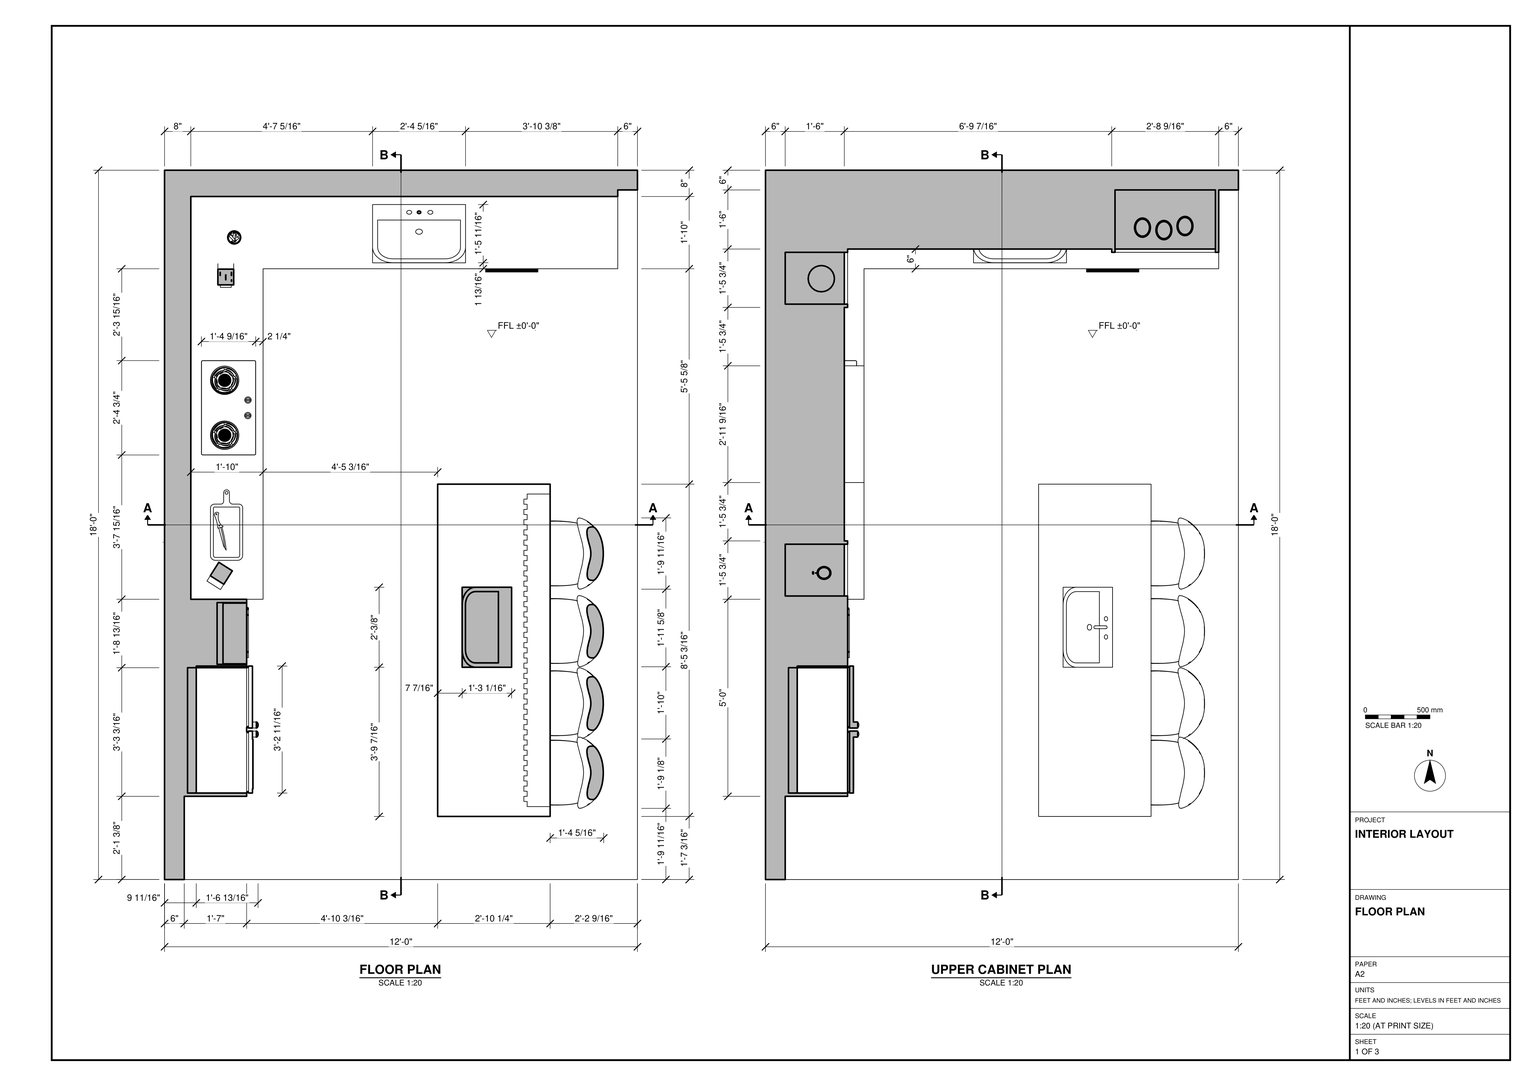
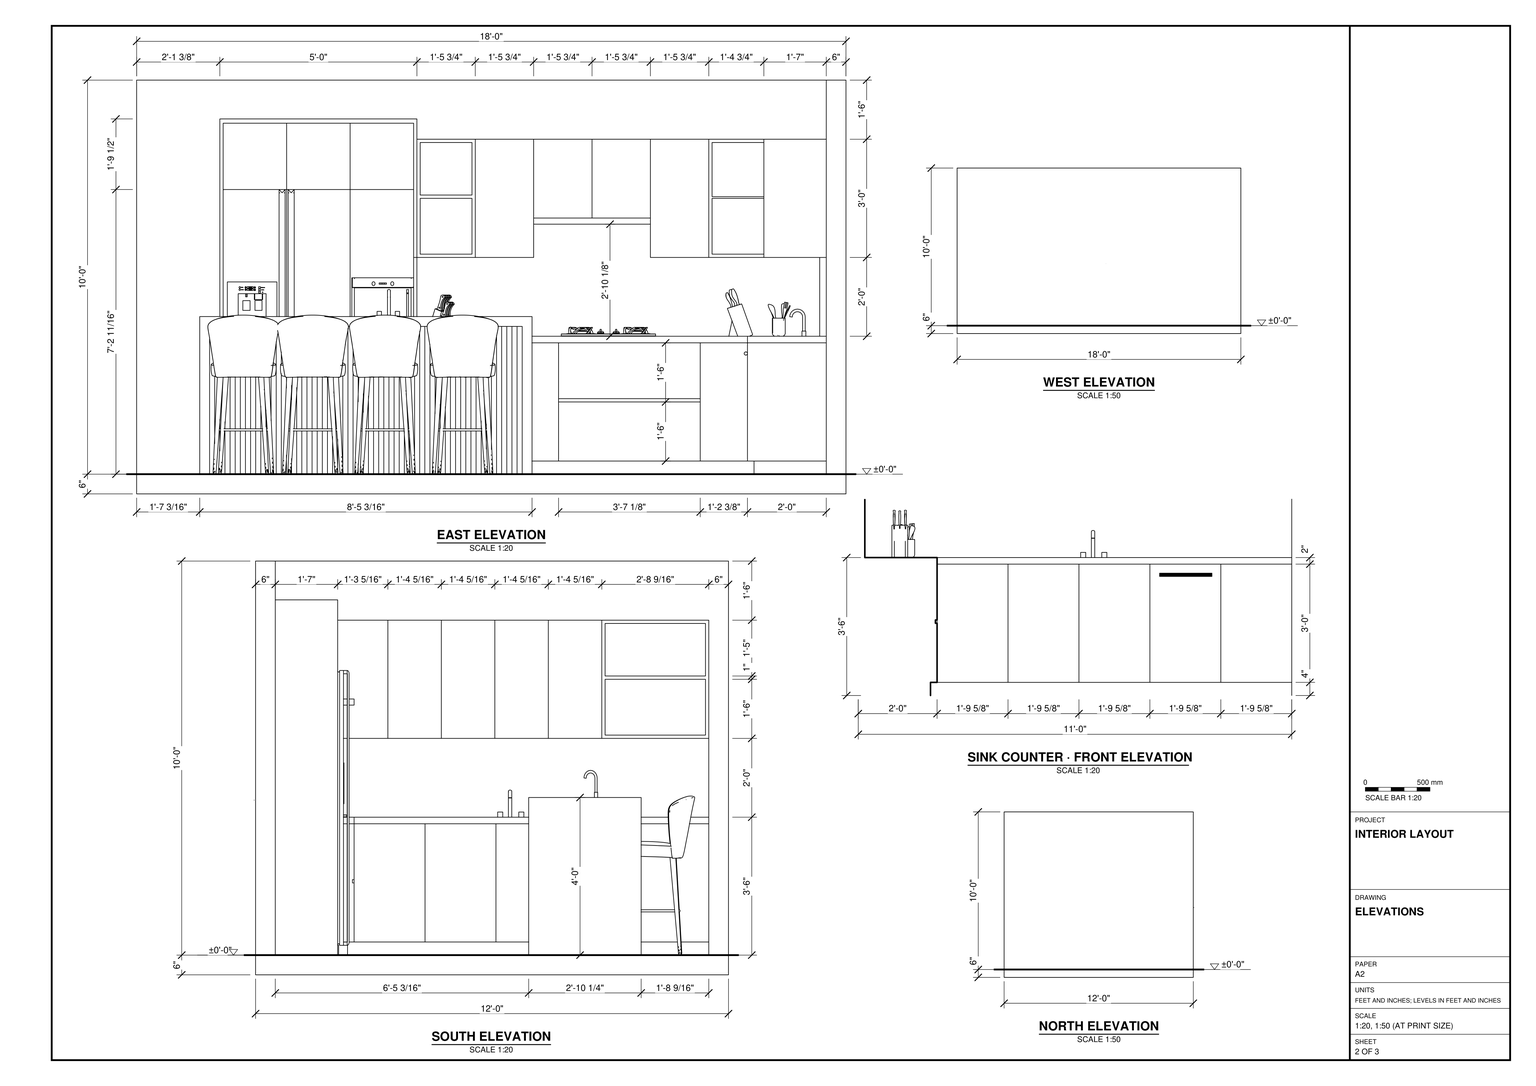
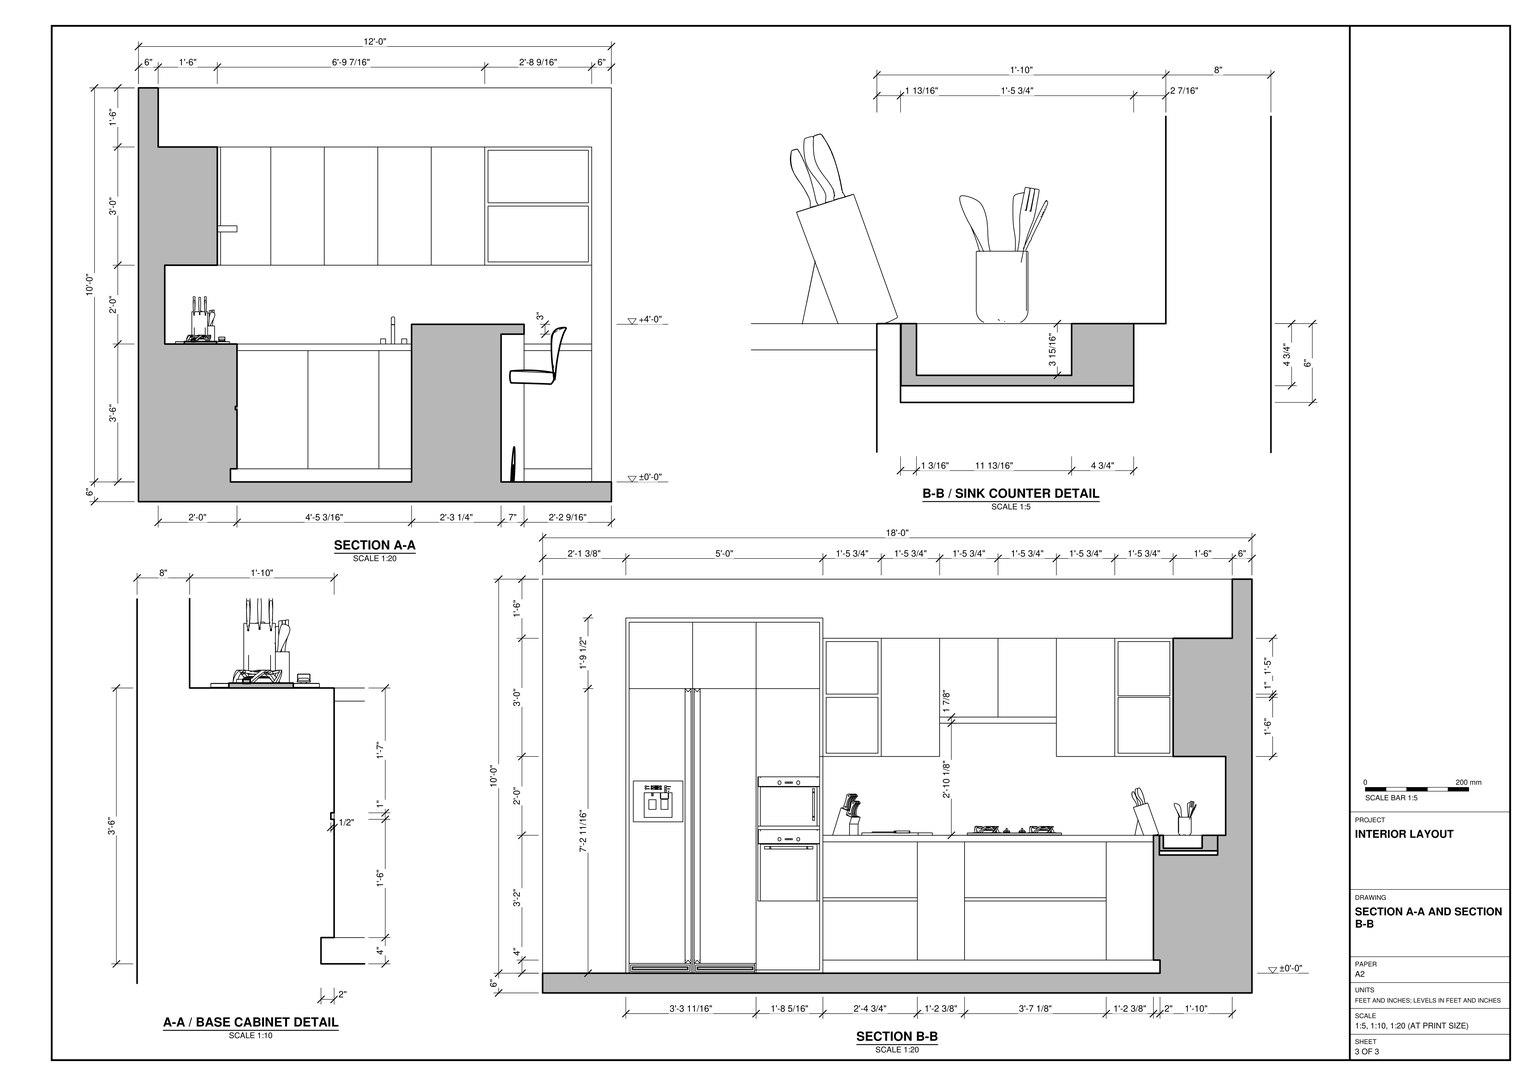
Build the kitchen interior in SketchUp from task_files/diagram_01.pdf. Work in feet and inches. Set the finished floor at ±0'-0". The overall model is 12'-0" wide by 18'-0" long and 10'-6" high, including the 6" floor slab below the finished floor. Model the north and west walls at their drawn thicknesses, rising 10'-0" above the floor. Leave the south and east sides open as shown.

Use the floor plan to lay out the tall appliance bank and cooktop along the west wall, with the counter turning the corner to the sink on the north wall. Model the base cabinet fronts, recessed toe kicks, worktops and sink recess. Use the upper cabinet plan for cabinet depths and the elevations for front divisions, stacked shelf bays and the raised clearance over the cooktop.

Place the freestanding island parallel to the west counter, leaving the working aisle shown in plan. Include the island sink and tap, the projecting counter edge and four seats along the east side. Use section A-A to set the island height and seating overhang. Appliances, decor and loose items may be any suitable library components. Keep each wall, slab, furniture piece and joinery unit in a separate group or component, and use components for repeated parts. Save one SketchUp model as output_files/l_shaped_kitchen_with_a_freestanding_sink_island.skp.

# SketchUp Ruby script. Lengths in inches.
U = 1.inch
M = Sketchup.active_model
def pt(a) = Geom::Point3d.new(a.map { |v| v * U })
def face(e, loops, mat)
  f = e.add_face(loops[0].map { |a| pt(a) })
  loops[1..].each { |l| e.add_face(l.map { |a| pt(a) }).erase! }
  f.material = f.back_material = mat if mat
  f
end
# faces: each face lists its corners as indices into pts; further lists are holes
def faces(e, pts, list, mat = nil) = list.each { |f| face(e, (f[0].is_a?(Array) ? f : [f]).map { |l| l.map { |i| pts[i] } }, mat) }
# xy, xz, yz: faces in a plane at the given z, y or x. An outline is a flat list of corners, or four numbers for a rectangle; further outlines are holes
def ring(l) = l.size == 4 ? [[l[0], l[1]], [l[2], l[1]], [l[2], l[3]], [l[0], l[3]]] : l.each_slice(2).to_a
def flat(e, list, mat, &to3) = list.each { |f| face(e, (f[0].is_a?(Array) ? f : [f]).map { |l| ring(l).map { |u, v| to3.(u, v) } }, mat) }
def xy(e, z, list, mat = nil) = flat(e, list, mat) { |x, y| [x, y, z] }
def xz(e, y, list, mat = nil) = flat(e, list, mat) { |x, z| [x, y, z] }
def yz(e, x, list, mat = nil) = flat(e, list, mat) { |y, z| [x, y, z] }
def lines(e, pts, list) = list.each { |a, b| e.add_line(pt(pts[a]), pt(pts[b])) }
# prism: a flat outline (further loops are holes) pulled along v
def prism(e, loops, v, mat = nil)
  f = face(e, loops, mat); d = Geom::Vector3d.new(v.map { |x| x * U })
  f.pushpull(f.normal.samedirection?(d) ? d.length : -d.length)
end
def box(e, o, s, mat = nil) = prism(e, [[o, [o[0] + s[0], o[1], o[2]], [o[0] + s[0], o[1] + s[1], o[2]], [o[0], o[1] + s[1], o[2]]]], [0, 0, s[2]], mat)
def at(x, y, z, deg = 0) = Geom::Transformation.translation(pt([x, y, z])) * Geom::Transformation.rotation(ORIGIN, Z_AXIS, deg.degrees)
def axes(o, x, y, z) = Geom::Transformation.new([*x, 0, *y, 0, *z, 0, *pt(o).to_a, 1])
def part(name) = M.definitions.add(name)
# library, detail: a bought-in or finely detailed component or shape, given as its bounding box
def library(name, o, s) = part(name).tap { |d| box(d.entities, o, s) }
def detail(e, o, s) = box(e.add_group.entities, o, s)
def put(e, d, t, mat = nil) = e.add_instance(d, t).tap { |i| i.material = mat if mat }
def group(e, t, mat = nil) = e.add_group.tap { |g| g.transformation = t; g.material = mat if mat }.entities
root = M.entities
M.materials.add("[0131_Silver]").color = [192, 192, 192]
M.materials.add("[0136_Charcoal]").color = [35, 35, 35]
M.materials.add("[Carrera Marble]").color = [242, 242, 242]
M.materials.add("[Carrera Marble]1").color = [239, 211, 174]
M.materials["[Carrera Marble]1"].alpha = 0.94
M.materials.add("[Carrera Marble]2").color = [228, 167, 92]
M.materials.add("[Formica Laminate Light]").color = [236, 189, 140]
M.materials.add("[Translucent Glass Blue]").color = [251, 172, 3]
M.materials["[Translucent Glass Blue]"].alpha = 0.5
c1 = library("Grupo3\#1",[-2.41,-4.18,0],[4.82,8.16,14.49])
c2 = library("KITCHEN+ITEMS+(30)",[-0.14,0,0],[4.76,4.15,3.43])
c3 = library("UTENCILIOS",[-3.38,-3.35,0],[5.31,6.7,10.38])
c4 = library("KITCHEN+KNIFES",[-11.85,-0.97,-1.38],[30.4,24.23,12.79])
c5 = library("KITCHEN+ITEMS+(3)",[-2.27,-9.02,0],[4.03,10.9,5.45])
c6 = library("Wash Basin simple",[0,0,0],[17.72,21.65,13])
c7 = library("GasStove_Black",[0,0,0],[28.74,16.54,2.72])
c8 = library("fridge",[0,-5.9,-2.99],[42,31.9,86.99])
c9 = library("bowls",[-48.35,57.53,67],[122.22,26.19,27.47])
c10 = library("Double oven",[0,0,0],[19.88,22.8,39.15])
c11 = library("CHAIR+-+(60)",[-15.99,-1.42,0],[17.65,18.29,35.43])
xy(root,0,[[0,0,144,216]])
xy(root,6,[[7,26.34,25,64.51]])
xy(root,6,[[[6,0,144,0,144,210,138,210,138,188,28,188,28,85.34,25,85.34,25,25.34,6,25.34],[83.16,19.22,83.16,120.4,117.41,120.4,117.41,117.4,110.41,117.4,110.41,115.84,109.41,115.84,109.41,114.28,110.41,114.28,110.41,112.72,109.41,112.72,109.41,111.16,110.41,111.16,110.41,109.6,109.41,109.6,109.41,108.04,110.41,108.04,110.41,106.48,109.41,106.48,109.41,104.92,110.41,104.92,110.41,103.36,109.41,103.36,109.41,101.8,110.41,101.8,110.41,100.24,109.41,100.24,109.41,98.68,110.41,98.68,110.41,97.12,109.41,97.12,109.41,95.56,110.41,95.56,110.41,94,109.41,94,109.41,92.4375,110.41,92.4375,110.41,90.875,109.41,90.875,109.41,89.31,110.41,89.31,110.41,87.75,109.41,87.75,109.41,86.19,110.41,86.19,110.41,84.63,109.41,84.63,109.41,83.07,110.41,83.07,110.41,81.51,109.41,81.51,109.41,79.95,110.41,79.95,110.41,78.39,109.41,78.39,109.41,76.83,110.41,76.83,110.41,75.27,109.41,75.27,109.41,73.71,110.41,73.71,110.41,72.15,109.41,72.15,109.41,70.59,110.41,70.59,110.41,69.03,109.41,69.03,109.41,67.47,110.41,67.47,110.41,65.91,109.41,65.91,109.41,64.35,110.41,64.35,110.41,62.79,109.41,62.79,109.41,61.23,110.41,61.23,110.41,59.67,109.41,59.67,109.41,58.11,110.41,58.11,110.41,56.55,109.41,56.55,109.41,54.98,110.41,54.98,110.41,53.42,109.41,53.42,109.41,51.86,110.41,51.86,110.41,50.3,109.41,50.3,109.41,48.74,110.41,48.74,110.41,47.18,109.41,47.18,109.41,45.62,110.41,45.62,110.41,44.0625,109.41,44.0625,109.41,42.5,110.41,42.5,110.41,40.94,109.41,40.94,109.41,39.38,110.41,39.38,110.41,37.82,109.41,37.82,109.41,36.26,110.41,36.26,110.41,34.7,109.41,34.7,109.41,33.14,110.41,33.14,110.41,31.58,109.41,31.58,109.41,30.02,110.41,30.02,110.41,28.46,109.41,28.46,109.41,26.9,110.41,26.9,110.41,25.34,109.41,25.34,109.41,23.78,110.41,23.78,110.41,22.22,117.41,22.22,117.41,19.22]]],"[Formica Laminate Light]")
xy(root,10,[[28,85.34,30,188]])
xy(root,10,[[30,186,138,188]],"[Formica Laminate Light]")
xy(root,28,[[16,65.53,25,84.34]])
xy(root,28,[[29.5,85.34,30,114.1],[29.5,128.48,30,171.62]],"[0136_Charcoal]")
xy(root,29,[[29.5,85.34,30,114.1],[29.5,128.48,30,171.62]],"[0136_Charcoal]")
xy(root,42,[[63.34,187.8,91.66,205.55]],"[0136_Charcoal]")
xy(root,42.28,[[97.76,185.67,113.69,185.68]])
xy(root,43.22,[[97.76,185.32,113.69,185.33]])
xy(root,43.25,[[97.76,185.45,113.69,185.58]])
xy(root,48,[[[8,85.34,30,85.34,30,186,138,186,138,208,8,208],[63.34,187.8,91.66,205.55]]],"[Carrera Marble]1")
xy(root,49,[[90.62,64.65,105.68,89.02]],"[0136_Charcoal]")
xy(root,51,[[110.41,22.22,110.41,23.78,109.41,23.78,109.41,25.34,110.41,25.34,110.41,26.9,109.41,26.9,109.41,28.46,110.41,28.46,110.41,30.02,109.41,30.02,109.41,31.58,110.41,31.58,110.41,33.14,109.41,33.14,109.41,34.7,110.41,34.7,110.41,36.26,109.41,36.26,109.41,37.82,110.41,37.82,110.41,39.38,109.41,39.38,109.41,40.94,110.41,40.94,110.41,42.5,109.41,42.5,109.41,44.0625,110.41,44.0625,110.41,45.62,109.41,45.62,109.41,47.18,110.41,47.18,110.41,48.74,109.41,48.74,109.41,50.3,110.41,50.3,110.41,51.86,109.41,51.86,109.41,53.42,110.41,53.42,110.41,54.98,109.41,54.98,109.41,56.55,110.41,56.55,110.41,58.11,109.41,58.11,109.41,59.67,110.41,59.67,110.41,61.23,109.41,61.23,109.41,62.79,110.41,62.79,110.41,64.35,109.41,64.35,109.41,65.91,110.41,65.91,110.41,67.47,109.41,67.47,109.41,69.03,110.41,69.03,110.41,70.59,109.41,70.59,109.41,72.15,110.41,72.15,110.41,73.71,109.41,73.71,109.41,75.27,110.41,75.27,110.41,76.83,109.41,76.83,109.41,78.39,110.41,78.39,110.41,79.95,109.41,79.95,109.41,81.51,110.41,81.51,110.41,83.07,109.41,83.07,109.41,84.63,110.41,84.63,110.41,86.19,109.41,86.19,109.41,87.75,110.41,87.75,110.41,89.31,109.41,89.31,109.41,90.875,110.41,90.875,110.41,92.4375,109.41,92.4375,109.41,94,110.41,94,110.41,95.56,109.41,95.56,109.41,97.12,110.41,97.12,110.41,98.68,109.41,98.68,109.41,100.24,110.41,100.24,110.41,101.8,109.41,101.8,109.41,103.36,110.41,103.36,110.41,104.92,109.41,104.92,109.41,106.48,110.41,106.48,110.41,108.04,109.41,108.04,109.41,109.6,110.41,109.6,110.41,111.16,109.41,111.16,109.41,112.72,110.41,112.72,110.41,114.28,109.41,114.28,109.41,115.84,110.41,115.84,110.41,117.4,117.41,117.4,117.41,22.22]],"[Carrera Marble]")
xy(root,54,[[[83.16,19.22,117.41,120.4],[90.62,64.65,105.68,89.02]]],"[Carrera Marble]")
xy(root,65.8125,[[16,65.53,25,84.34]])
xy(root,72,[[8,85.34,8,120.9,24,120.9,24,103.12,25,103.12,25,85.34],[8,156.45,8,208,24,208,24,192,25,192,25,174.22,24,174.22,24,156.45],[105.43,191,105.43,192,24,192,24,208,138,208,138,191]],"[Carrera Marble]")
xy(root,73,[[6,86.34,24,102.12],[6,175.22,24,191],[106.43,192,137,210]])
xy(root,73,[[24,86.34,25,102.12],[24,175.22,25,191],[106.43,191,137,192]],"[Formica Laminate Light]")
xy(root,82.13,[[8,120.9,30,156.45]],"[0136_Charcoal]")
xy(root,84,[[24,120.9,30,156.45]],"[0136_Charcoal]")
xy(root,90,[[6,86.34,24,102.12],[6,175.22,24,191],[106.43,192,137,210]])
xy(root,90,[[24,86.34,25,102.12],[24,175.22,25,191],[106.43,191,137,192]],"[Formica Laminate Light]")
xy(root,90.5,[[6,175.22,24,191]])
xy(root,90.5,[[24,175.22,25,191]],"[Formica Laminate Light]")
xy(root,91,[[6,86.34,24,102.12],[106.43,192,137,210]])
xy(root,91,[[24,86.34,25,102.12],[106.43,191,137,192]],"[Formica Laminate Light]")
xy(root,92.68,[[7,26.34,25,64.51]])
xy(root,107,[[6,86.34,24,102.12],[6,175.22,24,191],[106.43,192,137,210]])
xy(root,107,[[24,86.34,25,102.12],[24,175.22,25,191],[106.43,191,137,192]],"[Formica Laminate Light]")
xy(root,108,[[6,85.34,25,85.34,25,103.12,24,103.12,24,174.22,25,174.22,25,192,105.43,192,105.43,191,138,191,138,210,6,210]],"[Carrera Marble]")
xy(root,114.1875,[[6,25.34,25,85.34]],"[Formica Laminate Light]")
xy(root,126,[[0,0,6,0,6,210,144,210,144,216,0,216]],"[0131_Silver]")
xz(root,0,[[0,0,144,0,144,6,6,6,6,126,0,126]],"[0131_Silver]")
xz(root,19.22,[[83.16,6,117.41,54]],"[Carrera Marble]")
xz(root,22.22,[[110.41,6,117.41,51]],"[Carrera Marble]")
xz(root,23.78,[[109.41,6,110.41,51]],"[Carrera Marble]2")
xz(root,25.34,[[109.41,6,110.41,51]],"[Carrera Marble]2")
xz(root,25.34,[[6,6,25,114.1875]],"[Formica Laminate Light]")
xz(root,26.34,[[7,6,25,92.68]])
xz(root,26.9,[[109.41,6,110.41,51]],"[Carrera Marble]2")
xz(root,28.46,[[109.41,6,110.41,51]],"[Carrera Marble]2")
xz(root,30.02,[[109.41,6,110.41,51]],"[Carrera Marble]2")
xz(root,31.58,[[109.41,6,110.41,51]],"[Carrera Marble]2")
xz(root,33.14,[[109.41,6,110.41,51]],"[Carrera Marble]2")
xz(root,34.7,[[109.41,6,110.41,51]],"[Carrera Marble]2")
xz(root,36.26,[[109.41,6,110.41,51]],"[Carrera Marble]2")
xz(root,37.82,[[109.41,6,110.41,51]],"[Carrera Marble]2")
xz(root,39.38,[[109.41,6,110.41,51]],"[Carrera Marble]2")
xz(root,40.94,[[109.41,6,110.41,51]],"[Carrera Marble]2")
xz(root,42.5,[[109.41,6,110.41,51]],"[Carrera Marble]2")
xz(root,44.0625,[[109.41,6,110.41,51]],"[Carrera Marble]2")
xz(root,45.62,[[109.41,6,110.41,51]],"[Carrera Marble]2")
xz(root,47.18,[[109.41,6,110.41,51]],"[Carrera Marble]2")
xz(root,48.74,[[109.41,6,110.41,51]],"[Carrera Marble]2")
xz(root,50.3,[[109.41,6,110.41,51]],"[Carrera Marble]2")
xz(root,51.86,[[109.41,6,110.41,51]],"[Carrera Marble]2")
xz(root,53.42,[[109.41,6,110.41,51]],"[Carrera Marble]2")
xz(root,54.98,[[109.41,6,110.41,51]],"[Carrera Marble]2")
xz(root,56.55,[[109.41,6,110.41,51]],"[Carrera Marble]2")
xz(root,58.11,[[109.41,6,110.41,51]],"[Carrera Marble]2")
xz(root,59.67,[[109.41,6,110.41,51]],"[Carrera Marble]2")
xz(root,61.23,[[109.41,6,110.41,51]],"[Carrera Marble]2")
xz(root,62.79,[[109.41,6,110.41,51]],"[Carrera Marble]2")
xz(root,64.35,[[109.41,6,110.41,51]],"[Carrera Marble]2")
xz(root,64.51,[[7,6,25,92.68]])
xz(root,64.65,[[90.62,49,105.68,54]],"[0136_Charcoal]")
xz(root,65.53,[[16,28,25,65.8125]],"[Formica Laminate Light]")
xz(root,65.91,[[109.41,6,110.41,51]],"[Carrera Marble]2")
xz(root,67.47,[[109.41,6,110.41,51]],"[Carrera Marble]2")
xz(root,69.03,[[109.41,6,110.41,51]],"[Carrera Marble]2")
xz(root,70.59,[[109.41,6,110.41,51]],"[Carrera Marble]2")
xz(root,72.15,[[109.41,6,110.41,51]],"[Carrera Marble]2")
xz(root,73.71,[[109.41,6,110.41,51]],"[Carrera Marble]2")
xz(root,75.27,[[109.41,6,110.41,51]],"[Carrera Marble]2")
xz(root,76.83,[[109.41,6,110.41,51]],"[Carrera Marble]2")
xz(root,78.39,[[109.41,6,110.41,51]],"[Carrera Marble]2")
xz(root,79.95,[[109.41,6,110.41,51]],"[Carrera Marble]2")
xz(root,81.51,[[109.41,6,110.41,51]],"[Carrera Marble]2")
xz(root,83.07,[[109.41,6,110.41,51]],"[Carrera Marble]2")
xz(root,84.34,[[16,28,25,46],[16,46,25,48]])
xz(root,84.34,[[16,48,25,65.8125]],"[Formica Laminate Light]")
xz(root,84.63,[[109.41,6,110.41,51]],"[Carrera Marble]2")
xz(root,85.34,[[25,46,30,48]],"[Carrera Marble]1")
xz(root,85.34,[[25,6,28,10],[25,10,30,10,30,28,29.5,28,29.5,29,30,29,30,46,25,46],[8,48,25,72],[6,108,25,114.1875]],"[Formica Laminate Light]")
xz(root,86.19,[[109.41,6,110.41,51]],"[Carrera Marble]2")
xz(root,86.34,[[6,73,24,90],[6,91,24,107]])
xz(root,86.34,[[24,73,25,90],[24,91,25,107]],"[Formica Laminate Light]")
xz(root,87.75,[[109.41,6,110.41,51]],"[Carrera Marble]2")
xz(root,89.02,[[90.62,49,105.68,54]],"[0136_Charcoal]")
xz(root,89.31,[[109.41,6,110.41,51]],"[Carrera Marble]2")
xz(root,90.875,[[109.41,6,110.41,51]],"[Carrera Marble]2")
xz(root,92.4375,[[109.41,6,110.41,51]],"[Carrera Marble]2")
xz(root,94,[[109.41,6,110.41,51]],"[Carrera Marble]2")
xz(root,95.56,[[109.41,6,110.41,51]],"[Carrera Marble]2")
xz(root,97.12,[[109.41,6,110.41,51]],"[Carrera Marble]2")
xz(root,98.68,[[109.41,6,110.41,51]],"[Carrera Marble]2")
xz(root,100.24,[[109.41,6,110.41,51]],"[Carrera Marble]2")
xz(root,101.8,[[109.41,6,110.41,51]],"[Carrera Marble]2")
xz(root,102.12,[[6,73,24,90],[6,91,24,107]])
xz(root,102.12,[[24,73,25,90],[24,91,25,107]],"[Formica Laminate Light]")
xz(root,103.12,[[24,72,25,108]],"[Formica Laminate Light]")
xz(root,103.36,[[109.41,6,110.41,51]],"[Carrera Marble]2")
xz(root,104.92,[[109.41,6,110.41,51]],"[Carrera Marble]2")
xz(root,106.48,[[109.41,6,110.41,51]],"[Carrera Marble]2")
xz(root,108.04,[[109.41,6,110.41,51]],"[Carrera Marble]2")
xz(root,109.6,[[109.41,6,110.41,51]],"[Carrera Marble]2")
xz(root,111.16,[[109.41,6,110.41,51]],"[Carrera Marble]2")
xz(root,112.72,[[109.41,6,110.41,51]],"[Carrera Marble]2")
xz(root,114.1,[[29.5,28,30,29]],"[0136_Charcoal]")
xz(root,114.28,[[109.41,6,110.41,51]],"[Carrera Marble]2")
xz(root,115.84,[[109.41,6,110.41,51]],"[Carrera Marble]2")
xz(root,117.4,[[110.41,6,117.41,51]],"[Carrera Marble]")
xz(root,120.4,[[83.16,6,117.41,54]],"[Carrera Marble]")
xz(root,120.9,[[24,82.13,30,84]],"[0136_Charcoal]")
xz(root,120.9,[[8,72,24,82.13]],"[Carrera Marble]")
xz(root,128.48,[[29.5,28,30,29]],"[0136_Charcoal]")
xz(root,156.45,[[24,82.13,30,84]],"[0136_Charcoal]")
xz(root,156.45,[[8,72,24,82.13]],"[Carrera Marble]")
xz(root,171.62,[[29.5,28,30,29]],"[0136_Charcoal]")
xz(root,174.22,[[24,72,25,108]],"[Formica Laminate Light]")
xz(root,175.22,[[6,73,24,90],[24,73,25,90],[6,90.5,24,107],[24,90.5,25,107]])
xz(root,186,[[30,46,138,48]],"[Carrera Marble]1")
xz(root,186,[[30,10,51.6,46],[51.6,10,73.2,46],[73.2,10,94.8,46],[94.8,10,116.4,46],[116.4,10,138,46]],"[Formica Laminate Light]")
xz(root,187.8,[[63.34,42,91.66,48]],"[0136_Charcoal]")
xz(root,188,[[28,6,138,10]],"[Formica Laminate Light]")
xz(root,191,[[6,73,24,90],[6,90.5,24,107]])
xz(root,191,[[[105.43,72,138,108],[106.43,73,137,90],[106.43,91,137,107]],[24,73,25,90],[24,90.5,25,107]],"[Formica Laminate Light]")
xz(root,192,[[25,72,40.29,108],[40.29,72,56.57,108],[56.57,72,72.86,108],[72.86,72,89.14,108],[89.14,72,105.43,108]],"[Carrera Marble]")
xz(root,192,[[106.43,73,137,90],[106.43,91,137,107]],"[Translucent Glass Blue]")
xz(root,205.55,[[63.34,42,91.66,48]])
xz(root,208,[[8,48,138,72]],"[Carrera Marble]1")
xz(root,210,[[106.43,73,137,90],[106.43,91,137,107]])
xz(root,210,[[138,6,144,6,144,126,6,126,6,108,138,108]],"[0131_Silver]")
xz(root,216,[[0,0,144,126]])
yz(root,0,[[0,0,216,126]])
yz(root,6,[[86.34,73,102.12,90],[175.22,73,191,90],[175.22,90.5,191,107],[86.34,91,102.12,107]])
yz(root,6,[[0,6,25.34,6,25.34,114.1875,85.34,114.1875,85.34,108,210,108,210,126,0,126]],"[0131_Silver]")
yz(root,7,[[26.34,6,64.51,92.68]])
yz(root,8,[[85.34,48,208,48,208,72,156.45,72,156.45,82.13,120.9,82.13,120.9,72,85.34,72]],"[Carrera Marble]1")
yz(root,16,[[65.53,28,84.34,65.8125]],"[Formica Laminate Light]")
yz(root,24,[[103.12,72,120.9,108],[156.45,72,174.22,108],[120.9,84,138.67,108],[138.67,84,156.45,108]],"[Carrera Marble]")
yz(root,24,[[86.34,73,102.12,90],[175.22,73,191,90],[175.22,90.5,191,107],[86.34,91,102.12,107]],"[Translucent Glass Blue]")
yz(root,25,[[64.51,7,65.01,92.68]])
yz(root,25,[[25.34,6,26.34,6,26.34,112.875,84.34,112.875,84.34,72,85.34,72,85.34,114.1875,25.34,114.1875],[64.51,6,85.34,6,85.34,72,84.34,72,84.34,7,64.51,7],[65.01,7,84.34,7,84.34,28,65.53,28,65.53,65.8125,84.34,65.8125,84.34,92.68,65.01,92.68],[[85.34,72,103.12,108],[86.34,73,102.12,90],[86.34,91,102.12,107]],[[174.22,72,192,108],[175.22,73,191,90],[175.22,90.5,191,107]],
  [26.34,92.68,45.68,112.875],[45.68,92.68,65.01,112.875],[65.01,92.68,84.34,112.875]],"[Formica Laminate Light]")
yz(root,28,[[85.34,6,188,10]],"[Formica Laminate Light]")
yz(root,29.5,[[85.34,28,114.1,29],[128.48,28,171.62,29]],"[0136_Charcoal]")
yz(root,30,[[120.9,82.13,156.45,84]],"[0136_Charcoal]")
yz(root,30,[[85.34,46,186,48]],"[Carrera Marble]1")
yz(root,30,[[85.34,10,114.1,28],[114.1,10,128.48,46],[128.48,10,171.62,28],[171.62,10,186,46],[85.34,29,114.1,46],
  [128.48,29,171.62,46]],"[Formica Laminate Light]")
yz(root,63.34,[[187.8,42,205.55,48]],"[0136_Charcoal]")
yz(root,83.16,[[19.22,6,120.4,54]],"[Carrera Marble]")
yz(root,90.62,[[64.65,49,89.02,54]],"[0136_Charcoal]")
yz(root,91.66,[[187.8,42,205.55,48]],"[0136_Charcoal]")
yz(root,97.76,[[185.55,42.25,185.42,42.26,185.34,42.28,185.29,42.3,185.18,42.37,185.09,42.46,185.03,42.58,185,42.7,185.01,42.83,185.04,42.96,185.11,43.07,185.14,43.09,185.21,43.16,185.32,43.22,185.33,43.22,185.45,43.25,185.58,43.25,185.66,43.22,185.71,43.21,185.82,43.14,185.91,43.04,185.97,42.93,186,42.8,185.99,42.67,185.96,42.55,185.89,42.44,185.79,42.35,185.68,42.28,185.67,42.28]])
yz(root,105.43,[[191,72,192,108]])
yz(root,105.68,[[64.65,49,89.02,54]])
yz(root,106.43,[[192,73,210,90],[192,91,210,107]])
yz(root,106.43,[[191,73,192,90],[191,91,192,107]],"[Formica Laminate Light]")
yz(root,109.41,[[23.78,6,25.34,51],[26.9,6,28.46,51],[30.02,6,31.58,51],[33.14,6,34.7,51],[36.26,6,37.82,51],
  [39.38,6,40.94,51],[42.5,6,44.0625,51],[45.62,6,47.18,51],[48.74,6,50.3,51],[51.86,6,53.42,51],
  [54.98,6,56.55,51],[58.11,6,59.67,51],[61.23,6,62.79,51],[64.35,6,65.91,51],[67.47,6,69.03,51],
  [70.59,6,72.15,51],[73.71,6,75.27,51],[76.83,6,78.39,51],[79.95,6,81.51,51],[83.07,6,84.63,51],
  [86.19,6,87.75,51],[89.31,6,90.875,51],[92.4375,6,94,51],[95.56,6,97.12,51],[98.68,6,100.24,51],
  [101.8,6,103.36,51],[104.92,6,106.48,51],[108.04,6,109.6,51],[111.16,6,112.72,51],[114.28,6,115.84,51]],"[Carrera Marble]2")
yz(root,110.41,[[22.22,6,23.78,51],[25.34,6,26.9,51],[28.46,6,30.02,51],[31.58,6,33.14,51],[34.7,6,36.26,51],
  [37.82,6,39.38,51],[40.94,6,42.5,51],[44.0625,6,45.62,51],[47.18,6,48.74,51],[50.3,6,51.86,51],
  [53.42,6,54.98,51],[56.55,6,58.11,51],[59.67,6,61.23,51],[62.79,6,64.35,51],[65.91,6,67.47,51],
  [69.03,6,70.59,51],[72.15,6,73.71,51],[75.27,6,76.83,51],[78.39,6,79.95,51],[81.51,6,83.07,51],
  [84.63,6,86.19,51],[87.75,6,89.31,51],[90.875,6,92.4375,51],[94,6,95.56,51],[97.12,6,98.68,51],
  [100.24,6,101.8,51],[103.36,6,104.92,51],[106.48,6,108.04,51],[109.6,6,111.16,51],[112.72,6,114.28,51],
  [115.84,6,117.4,51]],"[Carrera Marble]2")
yz(root,113.69,[[185.55,42.25,185.67,42.28,185.34,42.28,185.42,42.26],[185.34,42.28,185.68,42.28,185.79,42.35,185.89,42.44,185.96,42.55,185.99,42.67,186,42.8,185.97,42.93,185.91,43.04,185.82,43.14,185.71,43.21,185.66,43.22,185.32,43.22,185.21,43.16,185.14,43.09,185.11,43.07,185.04,42.96,185.01,42.83,185,42.7,185.03,42.58,185.09,42.46,185.18,42.37,185.29,42.3],[185.33,43.22,185.66,43.22,185.58,43.25,185.45,43.25]])
yz(root,117.41,[[19.22,6,22.22,6,22.22,51,117.4,51,117.4,6,120.4,6,120.4,54,19.22,54]],"[Carrera Marble]")
yz(root,137,[[192,73,210,90],[192,91,210,107]])
yz(root,137,[[191,73,192,90],[191,91,192,107]],"[Formica Laminate Light]")
yz(root,138,[[191,72,210,108]],"[Carrera Marble]")
yz(root,138,[[186,46,210,48],[208,48,210,72]],"[Carrera Marble]1")
yz(root,138,[[188,6,210,10],[186,10,210,46]],"[Formica Laminate Light]")
yz(root,144,[[0,0,216,0,216,126,210,126,210,6,0,6]],"[0131_Silver]")
p = [[97.76,185.18,42.37],[97.76,185.29,42.3],[113.69,185.29,42.3],[113.69,185.18,42.37],[97.76,185.34,42.28],[97.76,185.42,42.26],
  [113.69,185.42,42.26],[113.69,185.34,42.28],[97.76,185.55,42.25],[113.69,185.55,42.25],[97.76,185.67,42.28],[113.69,185.67,42.28],
  [97.76,185.68,42.28],[97.76,185.79,42.35],[113.69,185.79,42.35],[113.69,185.68,42.28],[97.76,185.89,42.44],[113.69,185.89,42.44],
  [97.76,185.09,42.46],[97.76,185.14,42.41],[113.69,185.14,42.41],[113.69,185.09,42.46],[97.76,185.96,42.55],[113.69,185.96,42.55],
  [97.76,185.03,42.58],[113.69,185.03,42.58],[97.76,185.99,42.67],[113.69,185.99,42.67],[97.76,185,42.7],[113.69,185,42.7],
  [97.76,185.01,42.83],[113.69,185.01,42.83],[97.76,186,42.8],[113.69,186,42.8],[97.76,185.04,42.96],[113.69,185.04,42.96],
  [97.76,185.97,42.93],[113.69,185.97,42.93],[97.76,185.91,43.04],[113.69,185.91,43.04],[97.76,185.11,43.07],[113.69,185.11,43.07],
  [97.76,185.82,43.14],[113.69,185.82,43.14],[97.76,185.21,43.16],[97.76,185.14,43.09],[113.69,185.14,43.09],[113.69,185.21,43.16],
  [97.76,185.71,43.21],[113.69,185.71,43.21],[97.76,185.32,43.22],[113.69,185.32,43.22],[97.76,185.45,43.25],[97.76,185.33,43.22],
  [113.69,185.33,43.22],[113.69,185.45,43.25],[97.76,185.66,43.22],[97.76,185.58,43.25],[113.69,185.58,43.25],[113.69,185.66,43.22]]
faces(root,p,[[0,1,2,3],[4,5,6,7],[1,4,7,2],[5,8,9,6],[8,10,11,9],[12,13,14,15],[13,16,17,14],[18,19,20,21],
  [19,0,3,20],[16,22,23,17],[24,18,21,25],[22,26,27,23],[28,24,25,29],[30,28,29,31],[26,32,33,27],[34,30,31,35],
  [32,36,37,33],[36,38,39,37],[40,34,35,41],[38,42,43,39],[44,45,46,47],[45,40,41,46],[42,48,49,43],[50,44,47,51],
  [52,53,54,55],[56,57,58,59],[48,56,59,49]])
put(root,c1,at(18.65,183.59,47.94))
put(root,c2,axes([13.24,90.1,90.91],[1.72,0,0],[0,1.59,0],[0,0,2.35]))
put(root,c3,at(21.34,195.66,48))
put(root,c4,at(22.82,100.15,49.375,90))
put(root,c5,axes([17.21,98.66,73],[2,0,0],[0,1.30928,0],[0,0,1.494]))
put(root,c5,axes([127.37,197.77,91],[0,-2.0646,0],[1.70982,0,0],[0,0,2]))
put(root,c6,axes([63.34,205.55,43.27],[0,-1,0],[1.30767,0,0],[0,0,1]))
put(root,c7,at(27.76,129.29,48,90))
put(root,c8,axes([25,26.34,8.98],[0,0.92063,0],[-0.59,0,0],[0,0,0.99641]))
put(root,c9,at(61.29,118.63,6))
put(root,c10,axes([25.55,84.34,28],[-0.39,0,0],[0,-0.82515,0],[0,0,0.96578]))
put(root,c6,axes([105.68,89.02,49.27],[-0.85019,0,0],[0,-1.12553,0],[0,0,1]))
put(root,c11,axes([114.05,23.71,6],[0,-1.22963,0],[1.1658,0,0],[0,0,1.3674]))
put(root,c11,axes([114.05,44.84,6],[0,-1.22963,0],[1.1658,0,0],[0,0,1.3674]))
put(root,c11,axes([114.05,66.84,6],[0,-1.22963,0],[1.1658,0,0],[0,0,1.3674]))
put(root,c11,axes([114.05,90.46,6],[0,-1.22963,0],[1.1658,0,0],[0,0,1.3674]))
